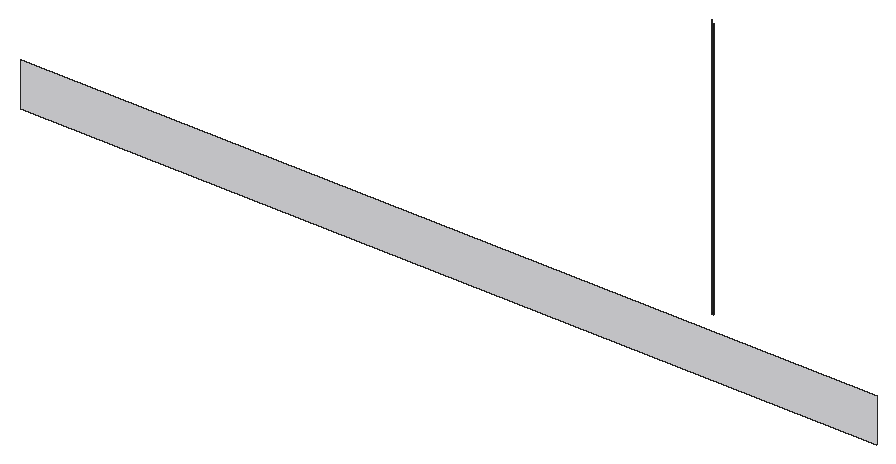
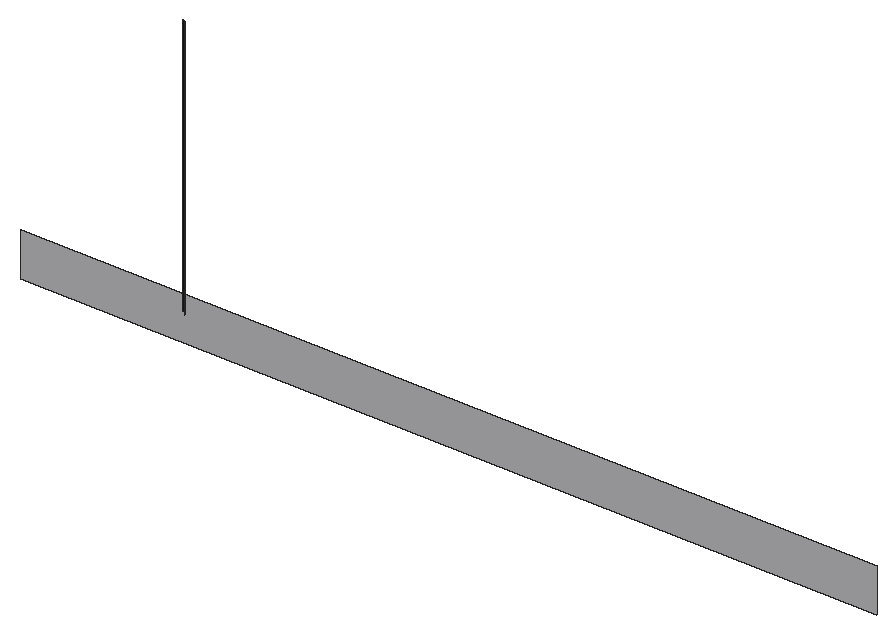
# SketchUp Ruby script. Lengths in inches.
U = 1.inch
M = Sketchup.active_model
def pt(a) = Geom::Point3d.new(a.map { |v| v * U })
def face(e, loops, mat)
  f = e.add_face(loops[0].map { |a| pt(a) })
  loops[1..].each { |l| e.add_face(l.map { |a| pt(a) }).erase! }
  f.material = f.back_material = mat if mat
  f
end
# faces: each face lists its corners as indices into pts; further lists are holes
def faces(e, pts, list, mat = nil) = list.each { |f| face(e, (f[0].is_a?(Array) ? f : [f]).map { |l| l.map { |i| pts[i] } }, mat) }
# xy, xz, yz: faces in a plane at the given z, y or x. An outline is a flat list of corners, or four numbers for a rectangle; further outlines are holes
def ring(l) = l.size == 4 ? [[l[0], l[1]], [l[2], l[1]], [l[2], l[3]], [l[0], l[3]]] : l.each_slice(2).to_a
def flat(e, list, mat, &to3) = list.each { |f| face(e, (f[0].is_a?(Array) ? f : [f]).map { |l| ring(l).map { |u, v| to3.(u, v) } }, mat) }
def xy(e, z, list, mat = nil) = flat(e, list, mat) { |x, y| [x, y, z] }
def xz(e, y, list, mat = nil) = flat(e, list, mat) { |x, z| [x, y, z] }
def yz(e, x, list, mat = nil) = flat(e, list, mat) { |y, z| [x, y, z] }
def lines(e, pts, list) = list.each { |a, b| e.add_line(pt(pts[a]), pt(pts[b])) }
# prism: a flat outline (further loops are holes) pulled along v
def prism(e, loops, v, mat = nil)
  f = face(e, loops, mat); d = Geom::Vector3d.new(v.map { |x| x * U })
  f.pushpull(f.normal.samedirection?(d) ? d.length : -d.length)
end
def box(e, o, s, mat = nil) = prism(e, [[o, [o[0] + s[0], o[1], o[2]], [o[0] + s[0], o[1] + s[1], o[2]], [o[0], o[1] + s[1], o[2]]]], [0, 0, s[2]], mat)
def at(x, y, z, deg = 0) = Geom::Transformation.translation(pt([x, y, z])) * Geom::Transformation.rotation(ORIGIN, Z_AXIS, deg.degrees)
def axes(o, x, y, z) = Geom::Transformation.new([*x, 0, *y, 0, *z, 0, *pt(o).to_a, 1])
def part(name) = M.definitions.add(name)
# library, detail: a bought-in or finely detailed component or shape, given as its bounding box
def library(name, o, s) = part(name).tap { |d| box(d.entities, o, s) }
def detail(e, o, s) = box(e.add_group.entities, o, s)
def put(e, d, t, mat = nil) = e.add_instance(d, t).tap { |i| i.material = mat if mat }
def group(e, t, mat = nil) = e.add_group.tap { |g| g.transformation = t; g.material = mat if mat }.entities
root = M.entities
M.materials.add("[0136_Charcoal]").color = [35, 35, 35]
M.materials.add("[Blinds Vertical Pattern]1").color = [239, 239, 242]
xz(root,225.17,[[189.02,137.875,283.04,142.6875]],"[Blinds Vertical Pattern]1")
p = [[263.05,227.61,142.6875],[263.28,227.52,142.6875],[263.28,227.52,171.3125],[263.05,227.61,171.3125],[262.86,227.76,142.6875],[262.86,227.76,171.3125],
  [262.71,227.96,142.6875],[262.71,227.96,171.3125]]
faces(root,p,[[0,1,2,3],[4,0,3,5],[6,4,5,7]],"[0136_Charcoal]")
